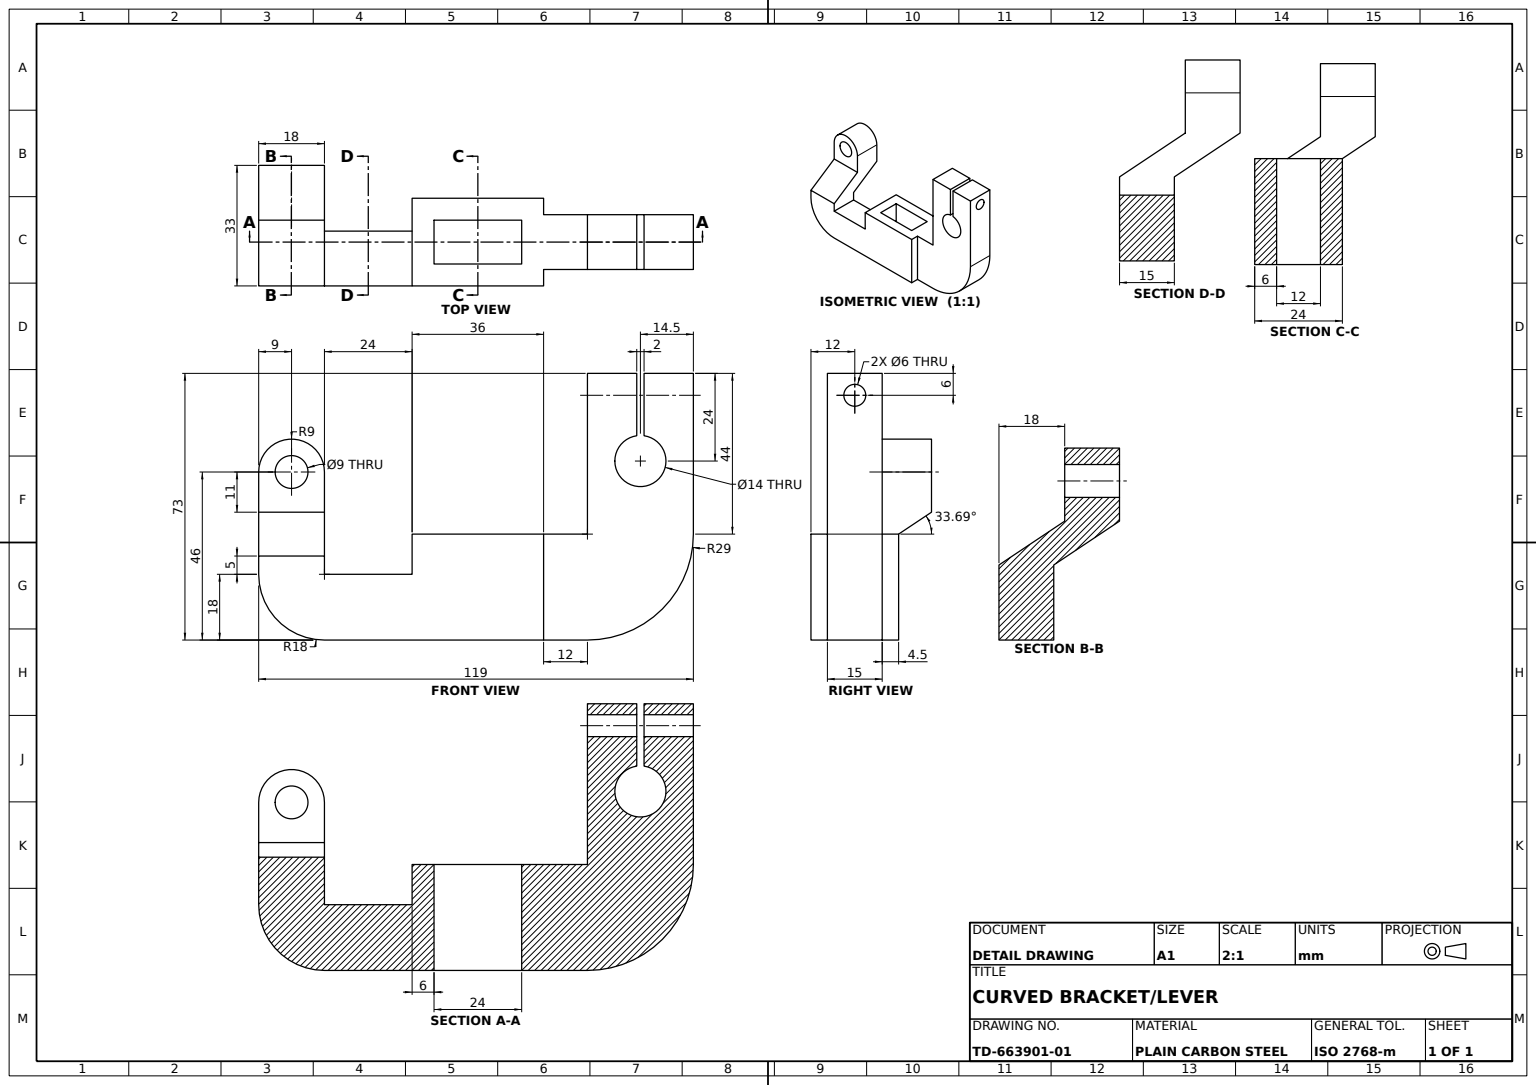
ISO-10303-21;
HEADER;
FILE_DESCRIPTION((''),'2;1');
FILE_NAME('','',(''),(''),'','','');
FILE_SCHEMA(('AUTOMOTIVE_DESIGN'));
ENDSEC;
DATA;
#1=APPLICATION_CONTEXT('');
#2=PRODUCT_CONTEXT('',#1,'mechanical');
#3=PRODUCT('','','',(#2));
#4=PRODUCT_DEFINITION_FORMATION('','',#3);
#5=PRODUCT_DEFINITION_CONTEXT('',#1,'design');
#6=PRODUCT_DEFINITION('','',#4,#5);
#7=PRODUCT_DEFINITION_SHAPE('','',#6);
#8=(LENGTH_UNIT()NAMED_UNIT(*)SI_UNIT(.MILLI.,.METRE.));
#9=(NAMED_UNIT(*)PLANE_ANGLE_UNIT()SI_UNIT($,.RADIAN.));
#10=(NAMED_UNIT(*)SI_UNIT($,.STERADIAN.)SOLID_ANGLE_UNIT());
#11=UNCERTAINTY_MEASURE_WITH_UNIT(LENGTH_MEASURE(1.E-05),#8,'distance_accuracy_value','');
#12=(GEOMETRIC_REPRESENTATION_CONTEXT(3)GLOBAL_UNCERTAINTY_ASSIGNED_CONTEXT((#11))GLOBAL_UNIT_ASSIGNED_CONTEXT((#8,#9,#10))REPRESENTATION_CONTEXT('',''));
#13=CARTESIAN_POINT('',(30.,52.5,-3.));
#14=VERTEX_POINT('',#13);
#15=CARTESIAN_POINT('',(30.,52.5,3.));
#16=VERTEX_POINT('',#15);
#17=CARTESIAN_POINT('',(30.,52.5,0.));
#18=DIRECTION('',(-1.,0.,0.));
#19=DIRECTION('',(0.,0.,1.));
#20=AXIS2_PLACEMENT_3D('',#17,#18,#19);
#21=CIRCLE('',#20,3.);
#22=EDGE_CURVE('',#14,#16,#21,.T.);
#23=ORIENTED_EDGE('',*,*,#22,.T.);
#24=CARTESIAN_POINT('',(43.5,52.5,3.));
#25=VERTEX_POINT('',#24);
#26=CARTESIAN_POINT('',(59.,52.5,3.));
#27=VECTOR('',#18,1000.);
#28=LINE('',#26,#27);
#29=EDGE_CURVE('',#25,#16,#28,.T.);
#30=ORIENTED_EDGE('',*,*,#29,.F.);
#31=CARTESIAN_POINT('',(43.5,52.5,-3.));
#32=VERTEX_POINT('',#31);
#33=CARTESIAN_POINT('',(43.5,52.5,0.));
#34=AXIS2_PLACEMENT_3D('',#33,#18,#19);
#35=CIRCLE('',#34,3.);
#36=EDGE_CURVE('',#32,#25,#35,.T.);
#37=ORIENTED_EDGE('',*,*,#36,.F.);
#38=CARTESIAN_POINT('',(59.,52.5,-3.));
#39=LINE('',#38,#27);
#40=EDGE_CURVE('',#32,#14,#39,.T.);
#41=ORIENTED_EDGE('',*,*,#40,.T.);
#42=EDGE_LOOP('',(#23,#30,#37,#41));
#43=FACE_OUTER_BOUND('',#42,.T.);
#44=CARTESIAN_POINT('',(59.,52.5,0.));
#45=AXIS2_PLACEMENT_3D('',#44,#18,#19);
#46=CYLINDRICAL_SURFACE('',#45,3.);
#47=ADVANCED_FACE('',(#43),#46,.F.);
#48=CARTESIAN_POINT('',(18.,-14.5,-12.));
#49=VERTEX_POINT('',#48);
#50=CARTESIAN_POINT('',(18.,14.5,-12.));
#51=VERTEX_POINT('',#50);
#52=DIRECTION('',(0.,1.,0.));
#53=VECTOR('',#52,1000.);
#54=LINE('',#48,#53);
#55=EDGE_CURVE('',#49,#51,#54,.T.);
#56=ORIENTED_EDGE('',*,*,#55,.T.);
#57=CARTESIAN_POINT('',(18.,14.5,-7.5));
#58=VERTEX_POINT('',#57);
#59=CARTESIAN_POINT('',(18.,14.5,12.));
#60=DIRECTION('',(0.,0.,-1.));
#61=VECTOR('',#60,1000.);
#62=LINE('',#59,#61);
#63=EDGE_CURVE('',#58,#51,#62,.T.);
#64=ORIENTED_EDGE('',*,*,#63,.F.);
#65=CARTESIAN_POINT('',(18.,-14.5,-7.5));
#66=VERTEX_POINT('',#65);
#67=LINE('',#65,#53);
#68=EDGE_CURVE('',#66,#58,#67,.T.);
#69=ORIENTED_EDGE('',*,*,#68,.F.);
#70=VECTOR('',#19,1000.);
#71=LINE('',#48,#70);
#72=EDGE_CURVE('',#49,#66,#71,.T.);
#73=ORIENTED_EDGE('',*,*,#72,.F.);
#74=EDGE_LOOP('',(#56,#64,#69,#73));
#75=FACE_OUTER_BOUND('',#74,.T.);
#76=AXIS2_PLACEMENT_3D('',#48,#18,#19);
#77=PLANE('',#76);
#78=ADVANCED_FACE('',(#75),#77,.F.);
#79=CARTESIAN_POINT('',(-12.,-14.5,6.));
#80=VERTEX_POINT('',#79);
#81=CARTESIAN_POINT('',(12.,-14.5,6.));
#82=VERTEX_POINT('',#81);
#83=DIRECTION('',(1.,0.,0.));
#84=VECTOR('',#83,1000.);
#85=LINE('',#79,#84);
#86=EDGE_CURVE('',#80,#82,#85,.T.);
#87=ORIENTED_EDGE('',*,*,#86,.F.);
#88=CARTESIAN_POINT('',(-12.,14.5,6.));
#89=VERTEX_POINT('',#88);
#90=LINE('',#79,#53);
#91=EDGE_CURVE('',#80,#89,#90,.T.);
#92=ORIENTED_EDGE('',*,*,#91,.T.);
#93=CARTESIAN_POINT('',(12.,14.5,6.));
#94=VERTEX_POINT('',#93);
#95=CARTESIAN_POINT('',(-18.,14.5,6.));
#96=LINE('',#95,#27);
#97=EDGE_CURVE('',#94,#89,#96,.T.);
#98=ORIENTED_EDGE('',*,*,#97,.F.);
#99=LINE('',#81,#53);
#100=EDGE_CURVE('',#82,#94,#99,.T.);
#101=ORIENTED_EDGE('',*,*,#100,.F.);
#102=EDGE_LOOP('',(#87,#92,#98,#101));
#103=FACE_OUTER_BOUND('',#102,.T.);
#104=AXIS2_PLACEMENT_3D('',#79,#19,#83);
#105=PLANE('',#104);
#106=ADVANCED_FACE('',(#103),#105,.F.);
#107=CARTESIAN_POINT('',(45.5,41.428203,-7.5));
#108=VERTEX_POINT('',#107);
#109=CARTESIAN_POINT('',(45.5,58.5,-7.5));
#110=VERTEX_POINT('',#109);
#111=CARTESIAN_POINT('',(45.5,-14.5,-7.5));
#112=LINE('',#111,#53);
#113=EDGE_CURVE('',#108,#110,#112,.T.);
#114=ORIENTED_EDGE('',*,*,#113,.F.);
#115=CARTESIAN_POINT('',(45.5,41.428203,7.5));
#116=VERTEX_POINT('',#115);
#117=CARTESIAN_POINT('',(45.5,41.428203,-12.));
#118=LINE('',#117,#70);
#119=EDGE_CURVE('',#108,#116,#118,.T.);
#120=ORIENTED_EDGE('',*,*,#119,.T.);
#121=CARTESIAN_POINT('',(45.5,58.5,7.5));
#122=VERTEX_POINT('',#121);
#123=LINE('',#115,#53);
#124=EDGE_CURVE('',#116,#122,#123,.T.);
#125=ORIENTED_EDGE('',*,*,#124,.T.);
#126=CARTESIAN_POINT('',(45.5,58.5,-12.));
#127=LINE('',#126,#70);
#128=EDGE_CURVE('',#110,#122,#127,.T.);
#129=ORIENTED_EDGE('',*,*,#128,.F.);
#130=EDGE_LOOP('',(#114,#120,#125,#129));
#131=FACE_OUTER_BOUND('',#130,.T.);
#132=CARTESIAN_POINT('',(45.5,52.5,3.));
#133=VERTEX_POINT('',#132);
#134=CARTESIAN_POINT('',(45.5,52.5,-3.));
#135=VERTEX_POINT('',#134);
#136=CARTESIAN_POINT('',(45.5,52.5,0.));
#137=AXIS2_PLACEMENT_3D('',#136,#83,#60);
#138=CIRCLE('',#137,3.);
#139=EDGE_CURVE('',#133,#135,#138,.T.);
#140=ORIENTED_EDGE('',*,*,#139,.T.);
#141=EDGE_CURVE('',#135,#133,#138,.T.);
#142=ORIENTED_EDGE('',*,*,#141,.T.);
#143=EDGE_LOOP('',(#140,#142));
#144=FACE_BOUND('',#143,.T.);
#145=AXIS2_PLACEMENT_3D('',#117,#83,#60);
#146=PLANE('',#145);
#147=ADVANCED_FACE('',(#131,#144),#146,.F.);
#148=CARTESIAN_POINT('',(-60.,8.5,12.));
#149=VERTEX_POINT('',#148);
#150=CARTESIAN_POINT('',(-60.,20.5,-6.));
#151=VERTEX_POINT('',#150);
#152=DIRECTION('',(0.,0.554700196,-0.832050294));
#153=VECTOR('',#152,1000.);
#154=LINE('',#150,#153);
#155=EDGE_CURVE('',#149,#151,#154,.T.);
#156=ORIENTED_EDGE('',*,*,#155,.F.);
#157=CARTESIAN_POINT('',(-42.,8.5,12.));
#158=VERTEX_POINT('',#157);
#159=LINE('',#148,#27);
#160=EDGE_CURVE('',#158,#149,#159,.T.);
#161=ORIENTED_EDGE('',*,*,#160,.F.);
#162=CARTESIAN_POINT('',(-42.,20.5,-6.));
#163=VERTEX_POINT('',#162);
#164=LINE('',#162,#153);
#165=EDGE_CURVE('',#158,#163,#164,.T.);
#166=ORIENTED_EDGE('',*,*,#165,.T.);
#167=CARTESIAN_POINT('',(-1.775629,20.5,-6.));
#168=LINE('',#167,#27);
#169=EDGE_CURVE('',#163,#151,#168,.T.);
#170=ORIENTED_EDGE('',*,*,#169,.T.);
#171=EDGE_LOOP('',(#156,#161,#166,#170));
#172=FACE_OUTER_BOUND('',#171,.T.);
#173=DIRECTION('',(0.,0.832050294,0.554700196));
#174=DIRECTION('',(0.,-0.554700196,0.832050294));
#175=AXIS2_PLACEMENT_3D('',#167,#173,#174);
#176=PLANE('',#175);
#177=ADVANCED_FACE('',(#172),#176,.T.);
#178=CARTESIAN_POINT('',(59.,58.5,7.5));
#179=VERTEX_POINT('',#178);
#180=LINE('',#178,#27);
#181=EDGE_CURVE('',#179,#122,#180,.T.);
#182=ORIENTED_EDGE('',*,*,#181,.T.);
#183=ORIENTED_EDGE('',*,*,#124,.F.);
#184=CARTESIAN_POINT('',(51.5,34.5,7.5));
#185=VERTEX_POINT('',#184);
#186=CARTESIAN_POINT('',(44.5,34.5,7.5));
#187=AXIS2_PLACEMENT_3D('',#186,#19,#83);
#188=CIRCLE('',#187,7.);
#189=EDGE_CURVE('',#185,#116,#188,.T.);
#190=ORIENTED_EDGE('',*,*,#189,.F.);
#191=CARTESIAN_POINT('',(37.5,34.5,7.5));
#192=VERTEX_POINT('',#191);
#193=EDGE_CURVE('',#192,#185,#188,.T.);
#194=ORIENTED_EDGE('',*,*,#193,.F.);
#195=CARTESIAN_POINT('',(43.5,41.428203,7.5));
#196=VERTEX_POINT('',#195);
#197=EDGE_CURVE('',#196,#192,#188,.T.);
#198=ORIENTED_EDGE('',*,*,#197,.F.);
#199=CARTESIAN_POINT('',(43.5,58.5,7.5));
#200=VERTEX_POINT('',#199);
#201=DIRECTION('',(0.,-1.,0.));
#202=VECTOR('',#201,1000.);
#203=LINE('',#195,#202);
#204=EDGE_CURVE('',#200,#196,#203,.T.);
#205=ORIENTED_EDGE('',*,*,#204,.F.);
#206=CARTESIAN_POINT('',(30.,58.5,7.5));
#207=VERTEX_POINT('',#206);
#208=EDGE_CURVE('',#200,#207,#180,.T.);
#209=ORIENTED_EDGE('',*,*,#208,.T.);
#210=CARTESIAN_POINT('',(30.,14.5,7.5));
#211=VERTEX_POINT('',#210);
#212=LINE('',#210,#53);
#213=EDGE_CURVE('',#211,#207,#212,.T.);
#214=ORIENTED_EDGE('',*,*,#213,.F.);
#215=CARTESIAN_POINT('',(18.,14.5,7.5));
#216=VERTEX_POINT('',#215);
#217=CARTESIAN_POINT('',(-18.,14.5,7.5));
#218=LINE('',#217,#84);
#219=EDGE_CURVE('',#216,#211,#218,.T.);
#220=ORIENTED_EDGE('',*,*,#219,.F.);
#221=CARTESIAN_POINT('',(18.,-14.5,7.5));
#222=VERTEX_POINT('',#221);
#223=LINE('',#221,#53);
#224=EDGE_CURVE('',#222,#216,#223,.T.);
#225=ORIENTED_EDGE('',*,*,#224,.F.);
#226=CARTESIAN_POINT('',(30.,-14.5,7.5));
#227=VERTEX_POINT('',#226);
#228=CARTESIAN_POINT('',(59.,-14.5,7.5));
#229=LINE('',#228,#27);
#230=EDGE_CURVE('',#227,#222,#229,.T.);
#231=ORIENTED_EDGE('',*,*,#230,.F.);
#232=CARTESIAN_POINT('',(59.,14.5,7.5));
#233=VERTEX_POINT('',#232);
#234=AXIS2_PLACEMENT_3D('',#210,#60,#18);
#235=CIRCLE('',#234,29.);
#236=EDGE_CURVE('',#233,#227,#235,.T.);
#237=ORIENTED_EDGE('',*,*,#236,.F.);
#238=LINE('',#228,#53);
#239=EDGE_CURVE('',#233,#179,#238,.T.);
#240=ORIENTED_EDGE('',*,*,#239,.T.);
#241=EDGE_LOOP('',(#182,#183,#190,#194,#198,#205,#209,#214,#220,#225,#231,#237,#240));
#242=FACE_OUTER_BOUND('',#241,.T.);
#243=AXIS2_PLACEMENT_3D('',#228,#60,#18);
#244=PLANE('',#243);
#245=ADVANCED_FACE('',(#242),#244,.F.);
#246=CARTESIAN_POINT('',(-12.,-14.5,-6.));
#247=VERTEX_POINT('',#246);
#248=CARTESIAN_POINT('',(-12.,14.5,-6.));
#249=VERTEX_POINT('',#248);
#250=LINE('',#246,#53);
#251=EDGE_CURVE('',#247,#249,#250,.T.);
#252=ORIENTED_EDGE('',*,*,#251,.T.);
#253=CARTESIAN_POINT('',(-12.,14.5,12.));
#254=LINE('',#253,#61);
#255=EDGE_CURVE('',#89,#249,#254,.T.);
#256=ORIENTED_EDGE('',*,*,#255,.F.);
#257=ORIENTED_EDGE('',*,*,#91,.F.);
#258=LINE('',#79,#70);
#259=EDGE_CURVE('',#247,#80,#258,.T.);
#260=ORIENTED_EDGE('',*,*,#259,.F.);
#261=EDGE_LOOP('',(#252,#256,#257,#260));
#262=FACE_OUTER_BOUND('',#261,.T.);
#263=AXIS2_PLACEMENT_3D('',#79,#18,#19);
#264=PLANE('',#263);
#265=ADVANCED_FACE('',(#262),#264,.F.);
#266=ORIENTED_EDGE('',*,*,#230,.T.);
#267=CARTESIAN_POINT('',(18.,-14.5,12.));
#268=VERTEX_POINT('',#267);
#269=LINE('',#267,#70);
#270=EDGE_CURVE('',#222,#268,#269,.T.);
#271=ORIENTED_EDGE('',*,*,#270,.T.);
#272=CARTESIAN_POINT('',(-42.,-14.5,12.));
#273=VERTEX_POINT('',#272);
#274=CARTESIAN_POINT('',(-18.,-14.5,12.));
#275=LINE('',#274,#84);
#276=EDGE_CURVE('',#273,#268,#275,.T.);
#277=ORIENTED_EDGE('',*,*,#276,.F.);
#278=CARTESIAN_POINT('',(-42.,-14.5,-3.));
#279=VERTEX_POINT('',#278);
#280=LINE('',#272,#61);
#281=EDGE_CURVE('',#273,#279,#280,.T.);
#282=ORIENTED_EDGE('',*,*,#281,.T.);
#283=CARTESIAN_POINT('',(-18.,-14.5,-3.));
#284=VERTEX_POINT('',#283);
#285=LINE('',#278,#84);
#286=EDGE_CURVE('',#279,#284,#285,.T.);
#287=ORIENTED_EDGE('',*,*,#286,.T.);
#288=CARTESIAN_POINT('',(-18.,-14.5,-12.));
#289=VERTEX_POINT('',#288);
#290=LINE('',#288,#61);
#291=EDGE_CURVE('',#284,#289,#290,.T.);
#292=ORIENTED_EDGE('',*,*,#291,.T.);
#293=LINE('',#48,#84);
#294=EDGE_CURVE('',#289,#49,#293,.T.);
#295=ORIENTED_EDGE('',*,*,#294,.T.);
#296=ORIENTED_EDGE('',*,*,#72,.T.);
#297=CARTESIAN_POINT('',(30.,-14.5,-7.5));
#298=VERTEX_POINT('',#297);
#299=LINE('',#65,#84);
#300=EDGE_CURVE('',#66,#298,#299,.T.);
#301=ORIENTED_EDGE('',*,*,#300,.T.);
#302=CARTESIAN_POINT('',(30.,-14.5,12.));
#303=LINE('',#302,#61);
#304=EDGE_CURVE('',#227,#298,#303,.T.);
#305=ORIENTED_EDGE('',*,*,#304,.F.);
#306=EDGE_LOOP('',(#266,#271,#277,#282,#287,#292,#295,#296,#301,#305));
#307=FACE_OUTER_BOUND('',#306,.T.);
#308=ORIENTED_EDGE('',*,*,#86,.T.);
#309=CARTESIAN_POINT('',(12.,-14.5,-6.));
#310=VERTEX_POINT('',#309);
#311=LINE('',#81,#61);
#312=EDGE_CURVE('',#82,#310,#311,.T.);
#313=ORIENTED_EDGE('',*,*,#312,.T.);
#314=LINE('',#246,#27);
#315=EDGE_CURVE('',#310,#247,#314,.T.);
#316=ORIENTED_EDGE('',*,*,#315,.T.);
#317=ORIENTED_EDGE('',*,*,#259,.T.);
#318=EDGE_LOOP('',(#308,#313,#316,#317));
#319=FACE_BOUND('',#318,.T.);
#320=AXIS2_PLACEMENT_3D('',#267,#52,#18);
#321=PLANE('',#320);
#322=ADVANCED_FACE('',(#307,#319),#321,.F.);
#323=CARTESIAN_POINT('',(-46.5,31.5,-21.));
#324=VERTEX_POINT('',#323);
#325=CARTESIAN_POINT('',(-46.5,31.5,-6.));
#326=VERTEX_POINT('',#325);
#327=CARTESIAN_POINT('',(-46.5,31.5,-30.));
#328=LINE('',#327,#70);
#329=EDGE_CURVE('',#324,#326,#328,.T.);
#330=ORIENTED_EDGE('',*,*,#329,.F.);
#331=CARTESIAN_POINT('',(-55.5,31.5,-21.));
#332=VERTEX_POINT('',#331);
#333=CARTESIAN_POINT('',(-51.,31.5,-21.));
#334=AXIS2_PLACEMENT_3D('',#333,#60,#18);
#335=CIRCLE('',#334,4.5);
#336=EDGE_CURVE('',#324,#332,#335,.T.);
#337=ORIENTED_EDGE('',*,*,#336,.T.);
#338=CARTESIAN_POINT('',(-55.5,31.5,-6.));
#339=VERTEX_POINT('',#338);
#340=CARTESIAN_POINT('',(-55.5,31.5,-30.));
#341=LINE('',#340,#70);
#342=EDGE_CURVE('',#332,#339,#341,.T.);
#343=ORIENTED_EDGE('',*,*,#342,.T.);
#344=CARTESIAN_POINT('',(-51.,31.5,-6.));
#345=AXIS2_PLACEMENT_3D('',#344,#19,#83);
#346=CIRCLE('',#345,4.5);
#347=EDGE_CURVE('',#339,#326,#346,.T.);
#348=ORIENTED_EDGE('',*,*,#347,.T.);
#349=EDGE_LOOP('',(#330,#337,#343,#348));
#350=FACE_OUTER_BOUND('',#349,.T.);
#351=CARTESIAN_POINT('',(-51.,31.5,-30.));
#352=AXIS2_PLACEMENT_3D('',#351,#19,#83);
#353=CYLINDRICAL_SURFACE('',#352,4.5);
#354=ADVANCED_FACE('',(#350),#353,.F.);
#355=ORIENTED_EDGE('',*,*,#141,.F.);
#356=VERTEX_POINT('',#38);
#357=EDGE_CURVE('',#356,#135,#39,.T.);
#358=ORIENTED_EDGE('',*,*,#357,.F.);
#359=VERTEX_POINT('',#26);
#360=CIRCLE('',#45,3.);
#361=EDGE_CURVE('',#359,#356,#360,.T.);
#362=ORIENTED_EDGE('',*,*,#361,.F.);
#363=EDGE_CURVE('',#359,#133,#28,.T.);
#364=ORIENTED_EDGE('',*,*,#363,.T.);
#365=EDGE_LOOP('',(#355,#358,#362,#364));
#366=FACE_OUTER_BOUND('',#365,.T.);
#367=ADVANCED_FACE('',(#366),#46,.F.);
#368=CARTESIAN_POINT('',(43.5,41.428203,-7.5));
#369=VERTEX_POINT('',#368);
#370=CARTESIAN_POINT('',(43.5,41.428203,-12.));
#371=LINE('',#370,#70);
#372=EDGE_CURVE('',#369,#196,#371,.T.);
#373=ORIENTED_EDGE('',*,*,#372,.F.);
#374=CARTESIAN_POINT('',(43.5,58.5,-7.5));
#375=VERTEX_POINT('',#374);
#376=CARTESIAN_POINT('',(43.5,-14.5,-7.5));
#377=LINE('',#376,#202);
#378=EDGE_CURVE('',#375,#369,#377,.T.);
#379=ORIENTED_EDGE('',*,*,#378,.F.);
#380=CARTESIAN_POINT('',(43.5,58.5,-12.));
#381=LINE('',#380,#70);
#382=EDGE_CURVE('',#375,#200,#381,.T.);
#383=ORIENTED_EDGE('',*,*,#382,.T.);
#384=ORIENTED_EDGE('',*,*,#204,.T.);
#385=EDGE_LOOP('',(#373,#379,#383,#384));
#386=FACE_OUTER_BOUND('',#385,.T.);
#387=EDGE_CURVE('',#25,#32,#35,.T.);
#388=ORIENTED_EDGE('',*,*,#387,.T.);
#389=ORIENTED_EDGE('',*,*,#36,.T.);
#390=EDGE_LOOP('',(#388,#389));
#391=FACE_BOUND('',#390,.T.);
#392=AXIS2_PLACEMENT_3D('',#370,#18,#19);
#393=PLANE('',#392);
#394=ADVANCED_FACE('',(#386,#391),#393,.F.);
#395=CARTESIAN_POINT('',(-18.,14.5,-12.));
#396=VERTEX_POINT('',#395);
#397=LINE('',#395,#27);
#398=EDGE_CURVE('',#51,#396,#397,.T.);
#399=ORIENTED_EDGE('',*,*,#398,.F.);
#400=ORIENTED_EDGE('',*,*,#55,.F.);
#401=ORIENTED_EDGE('',*,*,#294,.F.);
#402=CARTESIAN_POINT('',(-18.,3.5,-12.));
#403=LINE('',#402,#202);
#404=EDGE_CURVE('',#396,#289,#403,.T.);
#405=ORIENTED_EDGE('',*,*,#404,.F.);
#406=EDGE_LOOP('',(#399,#400,#401,#405));
#407=FACE_OUTER_BOUND('',#406,.T.);
#408=CARTESIAN_POINT('',(30.,14.5,-12.));
#409=AXIS2_PLACEMENT_3D('',#408,#60,#18);
#410=PLANE('',#409);
#411=ADVANCED_FACE('',(#407),#410,.T.);
#412=CARTESIAN_POINT('',(-42.,20.5,-21.));
#413=VERTEX_POINT('',#412);
#414=CARTESIAN_POINT('',(-60.,20.5,-21.));
#415=VERTEX_POINT('',#414);
#416=CARTESIAN_POINT('',(-1.775629,20.5,-21.));
#417=LINE('',#416,#27);
#418=EDGE_CURVE('',#413,#415,#417,.T.);
#419=ORIENTED_EDGE('',*,*,#418,.T.);
#420=CARTESIAN_POINT('',(-60.,31.5,-21.));
#421=VERTEX_POINT('',#420);
#422=LINE('',#414,#202);
#423=EDGE_CURVE('',#421,#415,#422,.T.);
#424=ORIENTED_EDGE('',*,*,#423,.F.);
#425=CARTESIAN_POINT('',(-42.,31.5,-21.));
#426=VERTEX_POINT('',#425);
#427=AXIS2_PLACEMENT_3D('',#333,#19,#18);
#428=CIRCLE('',#427,9.);
#429=EDGE_CURVE('',#426,#421,#428,.T.);
#430=ORIENTED_EDGE('',*,*,#429,.F.);
#431=LINE('',#412,#202);
#432=EDGE_CURVE('',#426,#413,#431,.T.);
#433=ORIENTED_EDGE('',*,*,#432,.T.);
#434=EDGE_LOOP('',(#419,#424,#430,#433));
#435=FACE_OUTER_BOUND('',#434,.T.);
#436=EDGE_CURVE('',#332,#324,#335,.T.);
#437=ORIENTED_EDGE('',*,*,#436,.F.);
#438=ORIENTED_EDGE('',*,*,#336,.F.);
#439=EDGE_LOOP('',(#437,#438));
#440=FACE_BOUND('',#439,.T.);
#441=AXIS2_PLACEMENT_3D('',#416,#60,#18);
#442=PLANE('',#441);
#443=ADVANCED_FACE('',(#435,#440),#442,.T.);
#444=ORIENTED_EDGE('',*,*,#347,.F.);
#445=EDGE_CURVE('',#326,#339,#346,.T.);
#446=ORIENTED_EDGE('',*,*,#445,.F.);
#447=EDGE_LOOP('',(#444,#446));
#448=FACE_BOUND('',#447,.T.);
#449=ORIENTED_EDGE('',*,*,#169,.F.);
#450=CARTESIAN_POINT('',(-42.,31.5,-6.));
#451=VERTEX_POINT('',#450);
#452=LINE('',#162,#53);
#453=EDGE_CURVE('',#163,#451,#452,.T.);
#454=ORIENTED_EDGE('',*,*,#453,.T.);
#455=CARTESIAN_POINT('',(-60.,31.5,-6.));
#456=VERTEX_POINT('',#455);
#457=AXIS2_PLACEMENT_3D('',#344,#19,#18);
#458=CIRCLE('',#457,9.);
#459=EDGE_CURVE('',#451,#456,#458,.T.);
#460=ORIENTED_EDGE('',*,*,#459,.T.);
#461=LINE('',#150,#53);
#462=EDGE_CURVE('',#151,#456,#461,.T.);
#463=ORIENTED_EDGE('',*,*,#462,.F.);
#464=EDGE_LOOP('',(#449,#454,#460,#463));
#465=FACE_OUTER_BOUND('',#464,.T.);
#466=AXIS2_PLACEMENT_3D('',#167,#19,#83);
#467=PLANE('',#466);
#468=ADVANCED_FACE('',(#448,#465),#467,.T.);
#469=ORIENTED_EDGE('',*,*,#329,.T.);
#470=ORIENTED_EDGE('',*,*,#445,.T.);
#471=ORIENTED_EDGE('',*,*,#342,.F.);
#472=ORIENTED_EDGE('',*,*,#436,.T.);
#473=EDGE_LOOP('',(#469,#470,#471,#472));
#474=FACE_OUTER_BOUND('',#473,.T.);
#475=ADVANCED_FACE('',(#474),#353,.F.);
#476=CARTESIAN_POINT('',(59.,14.5,-7.5));
#477=VERTEX_POINT('',#476);
#478=CARTESIAN_POINT('',(59.,58.5,-7.5));
#479=VERTEX_POINT('',#478);
#480=CARTESIAN_POINT('',(59.,-14.5,-7.5));
#481=LINE('',#480,#53);
#482=EDGE_CURVE('',#477,#479,#481,.T.);
#483=ORIENTED_EDGE('',*,*,#482,.F.);
#484=CARTESIAN_POINT('',(30.,14.5,-7.5));
#485=AXIS2_PLACEMENT_3D('',#484,#19,#83);
#486=CIRCLE('',#485,29.);
#487=EDGE_CURVE('',#298,#477,#486,.T.);
#488=ORIENTED_EDGE('',*,*,#487,.F.);
#489=ORIENTED_EDGE('',*,*,#300,.F.);
#490=ORIENTED_EDGE('',*,*,#68,.T.);
#491=VERTEX_POINT('',#484);
#492=CARTESIAN_POINT('',(-18.,14.5,-7.5));
#493=LINE('',#492,#27);
#494=EDGE_CURVE('',#491,#58,#493,.T.);
#495=ORIENTED_EDGE('',*,*,#494,.F.);
#496=CARTESIAN_POINT('',(30.,58.5,-7.5));
#497=VERTEX_POINT('',#496);
#498=LINE('',#484,#202);
#499=EDGE_CURVE('',#497,#491,#498,.T.);
#500=ORIENTED_EDGE('',*,*,#499,.F.);
#501=CARTESIAN_POINT('',(18.,58.5,-7.5));
#502=LINE('',#501,#84);
#503=EDGE_CURVE('',#497,#375,#502,.T.);
#504=ORIENTED_EDGE('',*,*,#503,.T.);
#505=ORIENTED_EDGE('',*,*,#378,.T.);
#506=CARTESIAN_POINT('',(37.5,34.5,-7.5));
#507=VERTEX_POINT('',#506);
#508=CARTESIAN_POINT('',(44.5,34.5,-7.5));
#509=AXIS2_PLACEMENT_3D('',#508,#19,#83);
#510=CIRCLE('',#509,7.);
#511=EDGE_CURVE('',#369,#507,#510,.T.);
#512=ORIENTED_EDGE('',*,*,#511,.T.);
#513=CARTESIAN_POINT('',(51.5,34.5,-7.5));
#514=VERTEX_POINT('',#513);
#515=EDGE_CURVE('',#507,#514,#510,.T.);
#516=ORIENTED_EDGE('',*,*,#515,.T.);
#517=EDGE_CURVE('',#514,#108,#510,.T.);
#518=ORIENTED_EDGE('',*,*,#517,.T.);
#519=ORIENTED_EDGE('',*,*,#113,.T.);
#520=EDGE_CURVE('',#110,#479,#502,.T.);
#521=ORIENTED_EDGE('',*,*,#520,.T.);
#522=EDGE_LOOP('',(#483,#488,#489,#490,#495,#500,#504,#505,#512,#516,#518,#519,#521));
#523=FACE_OUTER_BOUND('',#522,.T.);
#524=AXIS2_PLACEMENT_3D('',#65,#19,#83);
#525=PLANE('',#524);
#526=ADVANCED_FACE('',(#523),#525,.F.);
#527=CARTESIAN_POINT('',(59.,58.5,12.));
#528=LINE('',#527,#61);
#529=EDGE_CURVE('',#179,#479,#528,.T.);
#530=ORIENTED_EDGE('',*,*,#529,.T.);
#531=ORIENTED_EDGE('',*,*,#520,.F.);
#532=ORIENTED_EDGE('',*,*,#128,.T.);
#533=ORIENTED_EDGE('',*,*,#181,.F.);
#534=EDGE_LOOP('',(#530,#531,#532,#533));
#535=FACE_OUTER_BOUND('',#534,.T.);
#536=CARTESIAN_POINT('',(30.,58.5,12.));
#537=AXIS2_PLACEMENT_3D('',#536,#201,#60);
#538=PLANE('',#537);
#539=ADVANCED_FACE('',(#535),#538,.F.);
#540=ORIENTED_EDGE('',*,*,#208,.F.);
#541=ORIENTED_EDGE('',*,*,#382,.F.);
#542=ORIENTED_EDGE('',*,*,#503,.F.);
#543=LINE('',#536,#61);
#544=EDGE_CURVE('',#207,#497,#543,.T.);
#545=ORIENTED_EDGE('',*,*,#544,.F.);
#546=EDGE_LOOP('',(#540,#541,#542,#545));
#547=FACE_OUTER_BOUND('',#546,.T.);
#548=ADVANCED_FACE('',(#547),#538,.F.);
#549=CARTESIAN_POINT('',(-60.,3.5,12.));
#550=VERTEX_POINT('',#549);
#551=CARTESIAN_POINT('',(-42.,3.5,12.));
#552=AXIS2_PLACEMENT_3D('',#551,#19,#18);
#553=CIRCLE('',#552,18.);
#554=EDGE_CURVE('',#550,#273,#553,.T.);
#555=ORIENTED_EDGE('',*,*,#554,.F.);
#556=CARTESIAN_POINT('',(-60.,3.5,-3.));
#557=VERTEX_POINT('',#556);
#558=CARTESIAN_POINT('',(-60.,3.5,-32.206164));
#559=LINE('',#558,#70);
#560=EDGE_CURVE('',#557,#550,#559,.T.);
#561=ORIENTED_EDGE('',*,*,#560,.F.);
#562=CARTESIAN_POINT('',(-42.,3.5,-3.));
#563=AXIS2_PLACEMENT_3D('',#562,#60,#83);
#564=CIRCLE('',#563,18.);
#565=EDGE_CURVE('',#279,#557,#564,.T.);
#566=ORIENTED_EDGE('',*,*,#565,.F.);
#567=ORIENTED_EDGE('',*,*,#281,.F.);
#568=EDGE_LOOP('',(#555,#561,#566,#567));
#569=FACE_OUTER_BOUND('',#568,.T.);
#570=CARTESIAN_POINT('',(-42.,3.5,-32.206164));
#571=AXIS2_PLACEMENT_3D('',#570,#19,#83);
#572=CYLINDRICAL_SURFACE('',#571,18.);
#573=ADVANCED_FACE('',(#569),#572,.T.);
#574=CARTESIAN_POINT('',(-18.,14.5,12.));
#575=VERTEX_POINT('',#574);
#576=CARTESIAN_POINT('',(-18.,3.5,12.));
#577=VERTEX_POINT('',#576);
#578=LINE('',#576,#202);
#579=EDGE_CURVE('',#575,#577,#578,.T.);
#580=ORIENTED_EDGE('',*,*,#579,.F.);
#581=LINE('',#574,#61);
#582=EDGE_CURVE('',#575,#396,#581,.T.);
#583=ORIENTED_EDGE('',*,*,#582,.T.);
#584=ORIENTED_EDGE('',*,*,#404,.T.);
#585=ORIENTED_EDGE('',*,*,#291,.F.);
#586=CARTESIAN_POINT('',(-18.,3.5,-3.));
#587=VERTEX_POINT('',#586);
#588=LINE('',#283,#53);
#589=EDGE_CURVE('',#284,#587,#588,.T.);
#590=ORIENTED_EDGE('',*,*,#589,.T.);
#591=LINE('',#576,#61);
#592=EDGE_CURVE('',#577,#587,#591,.T.);
#593=ORIENTED_EDGE('',*,*,#592,.F.);
#594=EDGE_LOOP('',(#580,#583,#584,#585,#590,#593));
#595=FACE_OUTER_BOUND('',#594,.T.);
#596=AXIS2_PLACEMENT_3D('',#576,#83,#60);
#597=PLANE('',#596);
#598=ADVANCED_FACE('',(#595),#597,.F.);
#599=CARTESIAN_POINT('',(59.,14.5,12.));
#600=LINE('',#599,#61);
#601=EDGE_CURVE('',#233,#477,#600,.T.);
#602=ORIENTED_EDGE('',*,*,#601,.T.);
#603=ORIENTED_EDGE('',*,*,#482,.T.);
#604=ORIENTED_EDGE('',*,*,#529,.F.);
#605=ORIENTED_EDGE('',*,*,#239,.F.);
#606=EDGE_LOOP('',(#602,#603,#604,#605));
#607=FACE_OUTER_BOUND('',#606,.T.);
#608=ORIENTED_EDGE('',*,*,#361,.T.);
#609=EDGE_CURVE('',#356,#359,#360,.T.);
#610=ORIENTED_EDGE('',*,*,#609,.T.);
#611=EDGE_LOOP('',(#608,#610));
#612=FACE_BOUND('',#611,.T.);
#613=AXIS2_PLACEMENT_3D('',#527,#18,#201);
#614=PLANE('',#613);
#615=ADVANCED_FACE('',(#607,#612),#614,.F.);
#616=ORIENTED_EDGE('',*,*,#357,.T.);
#617=ORIENTED_EDGE('',*,*,#139,.F.);
#618=ORIENTED_EDGE('',*,*,#363,.F.);
#619=ORIENTED_EDGE('',*,*,#609,.F.);
#620=EDGE_LOOP('',(#616,#617,#618,#619));
#621=FACE_OUTER_BOUND('',#620,.T.);
#622=ADVANCED_FACE('',(#621),#46,.F.);
#623=ORIENTED_EDGE('',*,*,#29,.T.);
#624=EDGE_CURVE('',#16,#14,#21,.T.);
#625=ORIENTED_EDGE('',*,*,#624,.T.);
#626=ORIENTED_EDGE('',*,*,#40,.F.);
#627=ORIENTED_EDGE('',*,*,#387,.F.);
#628=EDGE_LOOP('',(#623,#625,#626,#627));
#629=FACE_OUTER_BOUND('',#628,.T.);
#630=ADVANCED_FACE('',(#629),#46,.F.);
#631=ORIENTED_EDGE('',*,*,#432,.F.);
#632=LINE('',#425,#61);
#633=EDGE_CURVE('',#451,#426,#632,.T.);
#634=ORIENTED_EDGE('',*,*,#633,.F.);
#635=ORIENTED_EDGE('',*,*,#453,.F.);
#636=ORIENTED_EDGE('',*,*,#165,.F.);
#637=VERTEX_POINT('',#551);
#638=LINE('',#157,#53);
#639=EDGE_CURVE('',#637,#158,#638,.T.);
#640=ORIENTED_EDGE('',*,*,#639,.F.);
#641=VERTEX_POINT('',#562);
#642=LINE('',#551,#61);
#643=EDGE_CURVE('',#637,#641,#642,.T.);
#644=ORIENTED_EDGE('',*,*,#643,.T.);
#645=CARTESIAN_POINT('',(-42.,8.5,-3.));
#646=VERTEX_POINT('',#645);
#647=LINE('',#645,#202);
#648=EDGE_CURVE('',#646,#641,#647,.T.);
#649=ORIENTED_EDGE('',*,*,#648,.F.);
#650=VECTOR('',#174,1000.);
#651=LINE('',#645,#650);
#652=EDGE_CURVE('',#413,#646,#651,.T.);
#653=ORIENTED_EDGE('',*,*,#652,.F.);
#654=EDGE_LOOP('',(#631,#634,#635,#636,#640,#644,#649,#653));
#655=FACE_OUTER_BOUND('',#654,.T.);
#656=CARTESIAN_POINT('',(-42.,8.5,-32.206164));
#657=AXIS2_PLACEMENT_3D('',#656,#83,#60);
#658=PLANE('',#657);
#659=ADVANCED_FACE('',(#655),#658,.T.);
#660=LINE('',#420,#61);
#661=EDGE_CURVE('',#456,#421,#660,.T.);
#662=ORIENTED_EDGE('',*,*,#661,.F.);
#663=ORIENTED_EDGE('',*,*,#459,.F.);
#664=ORIENTED_EDGE('',*,*,#633,.T.);
#665=ORIENTED_EDGE('',*,*,#429,.T.);
#666=EDGE_LOOP('',(#662,#663,#664,#665));
#667=FACE_OUTER_BOUND('',#666,.T.);
#668=CARTESIAN_POINT('',(-51.,31.5,-41.124612));
#669=AXIS2_PLACEMENT_3D('',#668,#19,#83);
#670=CYLINDRICAL_SURFACE('',#669,9.);
#671=ADVANCED_FACE('',(#667),#670,.T.);
#672=ORIENTED_EDGE('',*,*,#515,.F.);
#673=CARTESIAN_POINT('',(37.5,34.5,-12.));
#674=LINE('',#673,#70);
#675=EDGE_CURVE('',#507,#192,#674,.T.);
#676=ORIENTED_EDGE('',*,*,#675,.T.);
#677=ORIENTED_EDGE('',*,*,#193,.T.);
#678=CARTESIAN_POINT('',(51.5,34.5,-12.));
#679=LINE('',#678,#70);
#680=EDGE_CURVE('',#514,#185,#679,.T.);
#681=ORIENTED_EDGE('',*,*,#680,.F.);
#682=EDGE_LOOP('',(#672,#676,#677,#681));
#683=FACE_OUTER_BOUND('',#682,.T.);
#684=CARTESIAN_POINT('',(44.5,34.5,-12.));
#685=AXIS2_PLACEMENT_3D('',#684,#19,#83);
#686=CYLINDRICAL_SURFACE('',#685,7.);
#687=ADVANCED_FACE('',(#683),#686,.F.);
#688=CARTESIAN_POINT('',(12.,14.5,-6.));
#689=VERTEX_POINT('',#688);
#690=LINE('',#309,#53);
#691=EDGE_CURVE('',#310,#689,#690,.T.);
#692=ORIENTED_EDGE('',*,*,#691,.T.);
#693=CARTESIAN_POINT('',(-18.,14.5,-6.));
#694=LINE('',#693,#84);
#695=EDGE_CURVE('',#249,#689,#694,.T.);
#696=ORIENTED_EDGE('',*,*,#695,.F.);
#697=ORIENTED_EDGE('',*,*,#251,.F.);
#698=ORIENTED_EDGE('',*,*,#315,.F.);
#699=EDGE_LOOP('',(#692,#696,#697,#698));
#700=FACE_OUTER_BOUND('',#699,.T.);
#701=AXIS2_PLACEMENT_3D('',#246,#60,#18);
#702=PLANE('',#701);
#703=ADVANCED_FACE('',(#700),#702,.F.);
#704=ORIENTED_EDGE('',*,*,#119,.F.);
#705=ORIENTED_EDGE('',*,*,#517,.F.);
#706=ORIENTED_EDGE('',*,*,#680,.T.);
#707=ORIENTED_EDGE('',*,*,#189,.T.);
#708=EDGE_LOOP('',(#704,#705,#706,#707));
#709=FACE_OUTER_BOUND('',#708,.T.);
#710=ADVANCED_FACE('',(#709),#686,.F.);
#711=ORIENTED_EDGE('',*,*,#270,.F.);
#712=ORIENTED_EDGE('',*,*,#224,.T.);
#713=VERTEX_POINT('',#59);
#714=EDGE_CURVE('',#713,#216,#62,.T.);
#715=ORIENTED_EDGE('',*,*,#714,.F.);
#716=LINE('',#267,#53);
#717=EDGE_CURVE('',#268,#713,#716,.T.);
#718=ORIENTED_EDGE('',*,*,#717,.F.);
#719=EDGE_LOOP('',(#711,#712,#715,#718));
#720=FACE_OUTER_BOUND('',#719,.T.);
#721=AXIS2_PLACEMENT_3D('',#267,#18,#19);
#722=PLANE('',#721);
#723=ADVANCED_FACE('',(#720),#722,.F.);
#724=ORIENTED_EDGE('',*,*,#372,.T.);
#725=ORIENTED_EDGE('',*,*,#197,.T.);
#726=ORIENTED_EDGE('',*,*,#675,.F.);
#727=ORIENTED_EDGE('',*,*,#511,.F.);
#728=EDGE_LOOP('',(#724,#725,#726,#727));
#729=FACE_OUTER_BOUND('',#728,.T.);
#730=ADVANCED_FACE('',(#729),#686,.F.);
#731=ORIENTED_EDGE('',*,*,#601,.F.);
#732=ORIENTED_EDGE('',*,*,#236,.T.);
#733=ORIENTED_EDGE('',*,*,#304,.T.);
#734=ORIENTED_EDGE('',*,*,#487,.T.);
#735=EDGE_LOOP('',(#731,#732,#733,#734));
#736=FACE_OUTER_BOUND('',#735,.T.);
#737=CARTESIAN_POINT('',(30.,14.5,12.));
#738=AXIS2_PLACEMENT_3D('',#737,#60,#18);
#739=CYLINDRICAL_SURFACE('',#738,29.);
#740=ADVANCED_FACE('',(#736),#739,.T.);
#741=ORIENTED_EDGE('',*,*,#554,.T.);
#742=ORIENTED_EDGE('',*,*,#276,.T.);
#743=ORIENTED_EDGE('',*,*,#717,.T.);
#744=LINE('',#59,#27);
#745=EDGE_CURVE('',#713,#575,#744,.T.);
#746=ORIENTED_EDGE('',*,*,#745,.T.);
#747=ORIENTED_EDGE('',*,*,#579,.T.);
#748=LINE('',#576,#27);
#749=EDGE_CURVE('',#577,#637,#748,.T.);
#750=ORIENTED_EDGE('',*,*,#749,.T.);
#751=ORIENTED_EDGE('',*,*,#639,.T.);
#752=ORIENTED_EDGE('',*,*,#160,.T.);
#753=LINE('',#549,#202);
#754=EDGE_CURVE('',#149,#550,#753,.T.);
#755=ORIENTED_EDGE('',*,*,#754,.T.);
#756=EDGE_LOOP('',(#741,#742,#743,#746,#747,#750,#751,#752,#755));
#757=FACE_OUTER_BOUND('',#756,.T.);
#758=PLANE('',#738);
#759=ADVANCED_FACE('',(#757),#758,.F.);
#760=ORIENTED_EDGE('',*,*,#100,.T.);
#761=CARTESIAN_POINT('',(12.,14.5,12.));
#762=LINE('',#761,#70);
#763=EDGE_CURVE('',#689,#94,#762,.T.);
#764=ORIENTED_EDGE('',*,*,#763,.F.);
#765=ORIENTED_EDGE('',*,*,#691,.F.);
#766=ORIENTED_EDGE('',*,*,#312,.F.);
#767=EDGE_LOOP('',(#760,#764,#765,#766));
#768=FACE_OUTER_BOUND('',#767,.T.);
#769=AXIS2_PLACEMENT_3D('',#81,#83,#60);
#770=PLANE('',#769);
#771=ADVANCED_FACE('',(#768),#770,.F.);
#772=CARTESIAN_POINT('',(-60.,8.5,-3.));
#773=VERTEX_POINT('',#772);
#774=LINE('',#772,#650);
#775=EDGE_CURVE('',#415,#773,#774,.T.);
#776=ORIENTED_EDGE('',*,*,#775,.F.);
#777=ORIENTED_EDGE('',*,*,#418,.F.);
#778=ORIENTED_EDGE('',*,*,#652,.T.);
#779=LINE('',#772,#84);
#780=EDGE_CURVE('',#773,#646,#779,.T.);
#781=ORIENTED_EDGE('',*,*,#780,.F.);
#782=EDGE_LOOP('',(#776,#777,#778,#781));
#783=FACE_OUTER_BOUND('',#782,.T.);
#784=CARTESIAN_POINT('',(-1.775629,8.5,-3.));
#785=DIRECTION('',(0.,-0.832050294,-0.554700196));
#786=AXIS2_PLACEMENT_3D('',#784,#785,#152);
#787=PLANE('',#786);
#788=ADVANCED_FACE('',(#783),#787,.T.);
#789=LINE('',#556,#53);
#790=EDGE_CURVE('',#557,#773,#789,.T.);
#791=ORIENTED_EDGE('',*,*,#790,.T.);
#792=ORIENTED_EDGE('',*,*,#780,.T.);
#793=ORIENTED_EDGE('',*,*,#648,.T.);
#794=LINE('',#586,#27);
#795=EDGE_CURVE('',#587,#641,#794,.T.);
#796=ORIENTED_EDGE('',*,*,#795,.F.);
#797=ORIENTED_EDGE('',*,*,#589,.F.);
#798=ORIENTED_EDGE('',*,*,#286,.F.);
#799=ORIENTED_EDGE('',*,*,#565,.T.);
#800=EDGE_LOOP('',(#791,#792,#793,#796,#797,#798,#799));
#801=FACE_OUTER_BOUND('',#800,.T.);
#802=AXIS2_PLACEMENT_3D('',#278,#19,#83);
#803=PLANE('',#802);
#804=ADVANCED_FACE('',(#801),#803,.F.);
#805=ORIENTED_EDGE('',*,*,#643,.F.);
#806=ORIENTED_EDGE('',*,*,#749,.F.);
#807=ORIENTED_EDGE('',*,*,#592,.T.);
#808=ORIENTED_EDGE('',*,*,#795,.T.);
#809=EDGE_LOOP('',(#805,#806,#807,#808));
#810=FACE_OUTER_BOUND('',#809,.T.);
#811=AXIS2_PLACEMENT_3D('',#576,#201,#83);
#812=PLANE('',#811);
#813=ADVANCED_FACE('',(#810),#812,.F.);
#814=ORIENTED_EDGE('',*,*,#462,.T.);
#815=ORIENTED_EDGE('',*,*,#661,.T.);
#816=ORIENTED_EDGE('',*,*,#423,.T.);
#817=ORIENTED_EDGE('',*,*,#775,.T.);
#818=ORIENTED_EDGE('',*,*,#790,.F.);
#819=ORIENTED_EDGE('',*,*,#560,.T.);
#820=ORIENTED_EDGE('',*,*,#754,.F.);
#821=ORIENTED_EDGE('',*,*,#155,.T.);
#822=EDGE_LOOP('',(#814,#815,#816,#817,#818,#819,#820,#821));
#823=FACE_OUTER_BOUND('',#822,.T.);
#824=AXIS2_PLACEMENT_3D('',#558,#18,#19);
#825=PLANE('',#824);
#826=ADVANCED_FACE('',(#823),#825,.T.);
#827=ORIENTED_EDGE('',*,*,#624,.F.);
#828=ORIENTED_EDGE('',*,*,#22,.F.);
#829=EDGE_LOOP('',(#827,#828));
#830=FACE_BOUND('',#829,.T.);
#831=ORIENTED_EDGE('',*,*,#544,.T.);
#832=ORIENTED_EDGE('',*,*,#499,.T.);
#833=LINE('',#737,#61);
#834=EDGE_CURVE('',#211,#491,#833,.T.);
#835=ORIENTED_EDGE('',*,*,#834,.F.);
#836=ORIENTED_EDGE('',*,*,#213,.T.);
#837=EDGE_LOOP('',(#831,#832,#835,#836));
#838=FACE_OUTER_BOUND('',#837,.T.);
#839=AXIS2_PLACEMENT_3D('',#737,#83,#60);
#840=PLANE('',#839);
#841=ADVANCED_FACE('',(#830,#838),#840,.F.);
#842=ORIENTED_EDGE('',*,*,#763,.T.);
#843=ORIENTED_EDGE('',*,*,#97,.T.);
#844=ORIENTED_EDGE('',*,*,#255,.T.);
#845=ORIENTED_EDGE('',*,*,#695,.T.);
#846=EDGE_LOOP('',(#842,#843,#844,#845));
#847=FACE_BOUND('',#846,.T.);
#848=ORIENTED_EDGE('',*,*,#398,.T.);
#849=ORIENTED_EDGE('',*,*,#582,.F.);
#850=ORIENTED_EDGE('',*,*,#745,.F.);
#851=ORIENTED_EDGE('',*,*,#714,.T.);
#852=ORIENTED_EDGE('',*,*,#219,.T.);
#853=ORIENTED_EDGE('',*,*,#834,.T.);
#854=ORIENTED_EDGE('',*,*,#494,.T.);
#855=ORIENTED_EDGE('',*,*,#63,.T.);
#856=EDGE_LOOP('',(#848,#849,#850,#851,#852,#853,#854,#855));
#857=FACE_OUTER_BOUND('',#856,.T.);
#858=AXIS2_PLACEMENT_3D('',#574,#201,#60);
#859=PLANE('',#858);
#860=ADVANCED_FACE('',(#847,#857),#859,.F.);
#861=CLOSED_SHELL('',(#47,#78,#106,#147,#177,#245,#265,#322,#354,#367,#394,#411,#443,#468,#475,#526,#539,#548,#573,#598,#615,#622,#630,#659,#671,#687,#703,#710,#723,#730,#740,#759,#771,#788,#804,#813,#826,#841,#860));
#862=MANIFOLD_SOLID_BREP('',#861);
#863=ADVANCED_BREP_SHAPE_REPRESENTATION('',(#862),#12);
#864=SHAPE_DEFINITION_REPRESENTATION(#7,#863);
ENDSEC;
END-ISO-10303-21;
